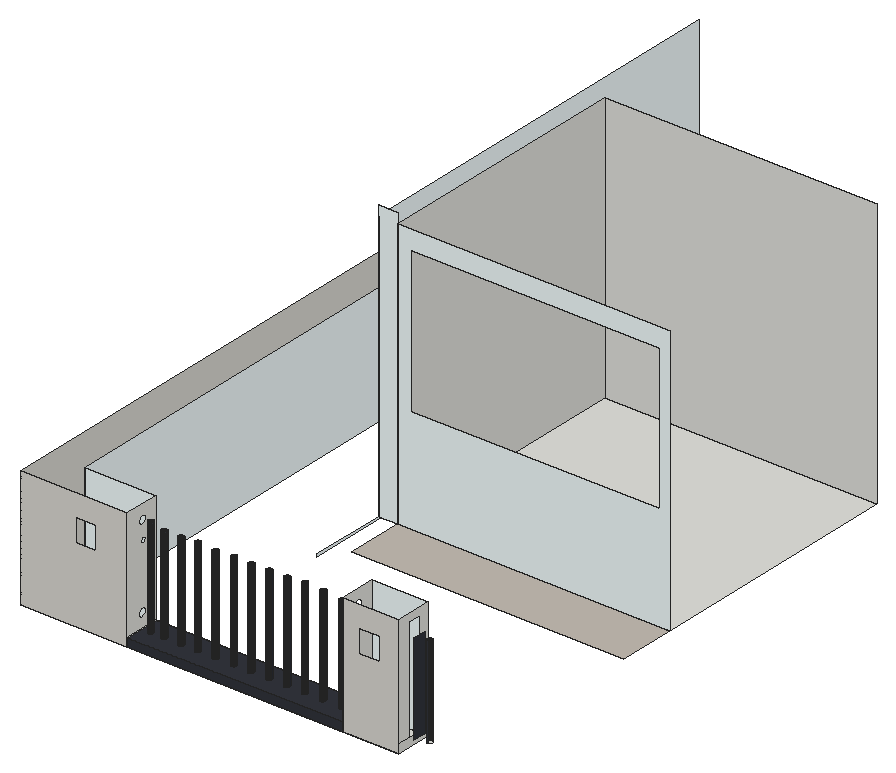
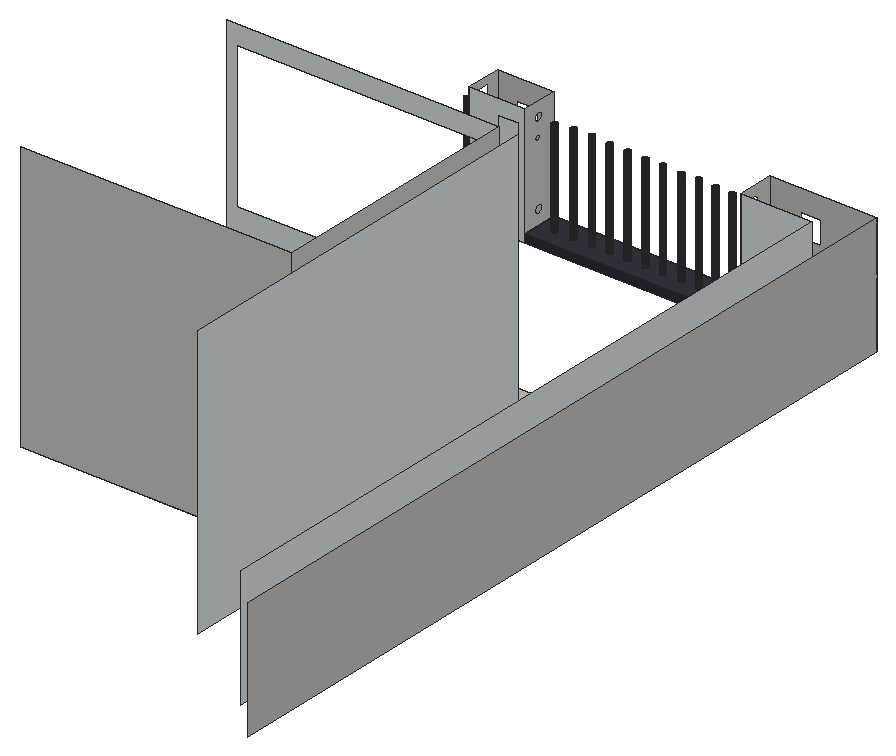
# SketchUp Ruby script. Lengths in inches.
U = 1.inch
M = Sketchup.active_model
def pt(a) = Geom::Point3d.new(a.map { |v| v * U })
def face(e, loops, mat)
  f = e.add_face(loops[0].map { |a| pt(a) })
  loops[1..].each { |l| e.add_face(l.map { |a| pt(a) }).erase! }
  f.material = f.back_material = mat if mat
  f
end
# faces: each face lists its corners as indices into pts; further lists are holes
def faces(e, pts, list, mat = nil) = list.each { |f| face(e, (f[0].is_a?(Array) ? f : [f]).map { |l| l.map { |i| pts[i] } }, mat) }
# xy, xz, yz: faces in a plane at the given z, y or x. An outline is a flat list of corners, or four numbers for a rectangle; further outlines are holes
def ring(l) = l.size == 4 ? [[l[0], l[1]], [l[2], l[1]], [l[2], l[3]], [l[0], l[3]]] : l.each_slice(2).to_a
def flat(e, list, mat, &to3) = list.each { |f| face(e, (f[0].is_a?(Array) ? f : [f]).map { |l| ring(l).map { |u, v| to3.(u, v) } }, mat) }
def xy(e, z, list, mat = nil) = flat(e, list, mat) { |x, y| [x, y, z] }
def xz(e, y, list, mat = nil) = flat(e, list, mat) { |x, z| [x, y, z] }
def yz(e, x, list, mat = nil) = flat(e, list, mat) { |y, z| [x, y, z] }
def lines(e, pts, list) = list.each { |a, b| e.add_line(pt(pts[a]), pt(pts[b])) }
# prism: a flat outline (further loops are holes) pulled along v
def prism(e, loops, v, mat = nil)
  f = face(e, loops, mat); d = Geom::Vector3d.new(v.map { |x| x * U })
  f.pushpull(f.normal.samedirection?(d) ? d.length : -d.length)
end
def box(e, o, s, mat = nil) = prism(e, [[o, [o[0] + s[0], o[1], o[2]], [o[0] + s[0], o[1] + s[1], o[2]], [o[0], o[1] + s[1], o[2]]]], [0, 0, s[2]], mat)
def at(x, y, z, deg = 0) = Geom::Transformation.translation(pt([x, y, z])) * Geom::Transformation.rotation(ORIGIN, Z_AXIS, deg.degrees)
def axes(o, x, y, z) = Geom::Transformation.new([*x, 0, *y, 0, *z, 0, *pt(o).to_a, 1])
def part(name) = M.definitions.add(name)
# library, detail: a bought-in or finely detailed component or shape, given as its bounding box
def library(name, o, s) = part(name).tap { |d| box(d.entities, o, s) }
def detail(e, o, s) = box(e.add_group.entities, o, s)
def put(e, d, t, mat = nil) = e.add_instance(d, t).tap { |i| i.material = mat if mat }
def group(e, t, mat = nil) = e.add_group.tap { |g| g.transformation = t; g.material = mat if mat }.entities
root = M.entities
M.materials.add("[Field Rectangle Tile]").color = [196, 189, 179]
M.materials.add("[Formica Laminate Dark]1").color = [50, 53, 60]
M.materials.add("[Terrazzo Tile Light]").color = [219, 217, 210]
M.materials.add("[White Subway Tile]").color = [243, 252, 253]
M.materials.add("[White Subway Tile]1").color = [243, 252, 253]
xy(root,0,[[383.65,0,1157.35,129.42],[1157.35,0,1357.59,129.42]])
xy(root,9,[[547.35,1008.89,1522.59,1933.89]])
xy(root,9,[[547.35,803.71,1522.59,1008.89]],"[Field Rectangle Tile]")
xy(root,29.875,[[416.3,55.58,413.8,55.72,411.41,56.51,409.31,57.89,407.64,59.76,406.51,62.01,405.99,64.47,406.14,66.98,406.92,69.36,408.3,71.46,410.18,73.14,412.42,74.27,414.88,74.78,417.39,74.64,419.77,73.85,421.875,72.47,423.55,70.6,424.68,68.35,425.19,65.89,425.05,63.38,424.26,61,422.88,58.9,421.01,57.22,418.76,56.09],[465.05,55.58,462.55,55.72,460.16,56.51,458.06,57.89,456.39,59.76,455.26,62.01,454.74,64.47,454.89,66.98,455.67,69.36,457.05,71.46,458.93,73.14,461.17,74.27,463.63,74.78,466.14,74.64,468.52,73.85,470.625,72.47,472.3,70.6,473.43,68.35,473.94,65.89,473.8,63.38,473.01,61,471.63,58.9,469.76,57.22,467.51,56.09],[525.12,55.58,522.61,55.72,520.22,56.51,518.12,57.89,516.45,59.76,515.32,62.01,514.81,64.47,514.95,66.98,515.74,69.36,517.11,71.46,518.99,73.14,521.23,74.27,523.69,74.78,526.2,74.64,528.59,73.85,530.6875,72.47,532.36,70.6,533.49,68.35,534,65.89,533.86,63.38,533.07,61,531.7,58.9,529.82,57.22,527.58,56.09],[585.24,55.58,582.73,55.72,580.35,56.51,578.25,57.89,576.57,59.76,575.44,62.01,574.93,64.47,575.07,66.98,575.86,69.36,577.24,71.46,579.11,73.14,581.36,74.27,583.82,74.78,586.33,74.64,588.71,73.85,590.8125,72.47,592.49,70.6,593.62,68.35,594.13,65.89,593.99,63.38,593.2,61,591.82,58.9,589.95,57.22,587.7,56.09],[648.8,55.58,646.3,55.72,643.91,56.51,641.81,57.89,640.14,59.76,639.01,62.01,638.49,64.47,638.64,66.98,639.42,69.36,640.8,71.46,642.68,73.14,644.92,74.27,647.38,74.78,649.89,74.64,652.27,73.85,654.375,72.47,656.05,70.6,657.18,68.35,657.69,65.89,657.55,63.38,656.76,61,655.38,58.9,653.51,57.22,651.26,56.09],
  [714.12,55.58,711.61,55.72,709.22,56.51,707.12,57.89,705.45,59.76,704.32,62.01,703.81,64.47,703.95,66.98,704.74,69.36,706.11,71.46,707.99,73.14,710.23,74.27,712.69,74.78,715.2,74.64,717.59,73.85,719.6875,72.47,721.36,70.6,722.49,68.35,723,65.89,722.86,63.38,722.07,61,720.7,58.9,718.82,57.22,716.58,56.09],[777.12,55.58,774.61,55.72,772.22,56.51,770.12,57.89,768.45,59.76,767.32,62.01,766.81,64.47,766.95,66.98,767.74,69.36,769.11,71.46,770.99,73.14,773.23,74.27,775.69,74.78,778.2,74.64,780.59,73.85,782.6875,72.47,784.36,70.6,785.49,68.35,786,65.89,785.86,63.38,785.07,61,783.7,58.9,781.82,57.22,779.58,56.09],[840.24,55.58,837.73,55.72,835.35,56.51,833.25,57.89,831.57,59.76,830.44,62.01,829.93,64.47,830.07,66.98,830.86,69.36,832.24,71.46,834.11,73.14,836.36,74.27,838.82,74.78,841.33,74.64,843.71,73.85,845.8125,72.47,847.49,70.6,848.62,68.35,849.13,65.89,848.99,63.38,848.2,61,846.82,58.9,844.95,57.22,842.7,56.09],[905.18,55.58,902.67,55.72,900.29,56.51,898.18,57.89,896.51,59.76,895.38,62.01,894.87,64.47,895.01,66.98,895.8,69.36,897.18,71.46,899.05,73.14,901.29,74.27,903.75,74.78,906.26,74.64,908.65,73.85,910.75,72.47,912.42,70.6,913.55,68.35,914.07,65.89,913.92,63.38,913.14,61,911.76,58.9,909.88,57.22,907.64,56.09],[968.99,55.58,966.48,55.72,964.1,56.51,962,57.89,960.32,59.76,959.19,62.01,958.68,64.47,958.82,66.98,959.61,69.36,960.99,71.46,962.86,73.14,965.11,74.27,967.57,74.78,970.08,74.64,972.46,73.85,974.5625,72.47,976.24,70.6,977.37,68.35,977.88,65.89,977.74,63.38,976.95,61,975.57,58.9,973.7,57.22,971.45,56.09],
  [1034.62,55.58,1032.11,55.72,1029.72,56.51,1027.62,57.89,1025.95,59.76,1024.82,62.01,1024.31,64.47,1024.45,66.98,1025.24,69.36,1026.61,71.46,1028.49,73.14,1030.73,74.27,1033.19,74.78,1035.7,74.64,1038.09,73.85,1040.1875,72.47,1041.86,70.6,1042.99,68.35,1043.5,65.89,1043.36,63.38,1042.57,61,1041.2,58.9,1039.32,57.22,1037.08,56.09],[1102.12,55.58,1099.61,55.72,1097.22,56.51,1095.12,57.89,1093.45,59.76,1092.32,62.01,1091.81,64.47,1091.95,66.98,1092.74,69.36,1094.11,71.46,1095.99,73.14,1098.23,74.27,1100.69,74.78,1103.2,74.64,1105.59,73.85,1107.6875,72.47,1109.36,70.6,1110.49,68.35,1111,65.89,1110.86,63.38,1110.07,61,1108.7,58.9,1106.82,57.22,1104.58,56.09],[1417.24,55.58,1414.73,55.72,1412.35,56.51,1410.25,57.89,1408.57,59.76,1407.44,62.01,1406.93,64.47,1407.07,66.98,1407.86,69.36,1409.24,71.46,1411.11,73.14,1413.36,74.27,1415.82,74.78,1418.33,74.64,1420.71,73.85,1422.8125,72.47,1424.49,70.6,1425.62,68.35,1426.13,65.89,1425.99,63.38,1425.2,61,1423.82,58.9,1421.95,57.22,1419.7,56.09]])
xy(root,29.875,[[[383.65,0,1157.35,129.42],[777.12,55.58,774.61,55.72,772.22,56.51,770.12,57.89,768.45,59.76,767.32,62.01,766.81,64.47,766.95,66.98,767.74,69.36,769.11,71.46,770.99,73.14,773.23,74.27,775.69,74.78,778.2,74.64,780.59,73.85,782.6875,72.47,784.36,70.6,785.49,68.35,786,65.89,785.86,63.38,785.07,61,783.7,58.9,781.82,57.22,779.58,56.09],[1102.12,55.58,1099.61,55.72,1097.22,56.51,1095.12,57.89,1093.45,59.76,1092.32,62.01,1091.81,64.47,1091.95,66.98,1092.74,69.36,1094.11,71.46,1095.99,73.14,1098.23,74.27,1100.69,74.78,1103.2,74.64,1105.59,73.85,1107.6875,72.47,1109.36,70.6,1110.49,68.35,1111,65.89,1110.86,63.38,1110.07,61,1108.7,58.9,1106.82,57.22,1104.58,56.09],[840.24,55.58,837.73,55.72,835.35,56.51,833.25,57.89,831.57,59.76,830.44,62.01,829.93,64.47,830.07,66.98,830.86,69.36,832.24,71.46,834.11,73.14,836.36,74.27,838.82,74.78,841.33,74.64,843.71,73.85,845.8125,72.47,847.49,70.6,848.62,68.35,849.13,65.89,848.99,63.38,848.2,61,846.82,58.9,844.95,57.22,842.7,56.09],[1034.62,55.58,1032.11,55.72,1029.72,56.51,1027.62,57.89,1025.95,59.76,1024.82,62.01,1024.31,64.47,1024.45,66.98,1025.24,69.36,1026.61,71.46,1028.49,73.14,1030.73,74.27,1033.19,74.78,1035.7,74.64,1038.09,73.85,1040.1875,72.47,1041.86,70.6,1042.99,68.35,1043.5,65.89,1043.36,63.38,1042.57,61,1041.2,58.9,1039.32,57.22,1037.08,56.09],[905.18,55.58,902.67,55.72,900.29,56.51,898.18,57.89,896.51,59.76,895.38,62.01,894.87,64.47,895.01,66.98,895.8,69.36,897.18,71.46,899.05,73.14,901.29,74.27,903.75,74.78,906.26,74.64,908.65,73.85,910.75,72.47,912.42,70.6,913.55,68.35,914.07,65.89,913.92,63.38,913.14,61,911.76,58.9,909.88,57.22,907.64,56.09],[968.99,55.58,966.48,55.72,964.1,56.51,962,57.89,960.32,59.76,959.19,62.01,958.68,64.47,958.82,66.98,959.61,69.36,960.99,71.46,962.86,73.14,965.11,74.27,967.57,74.78,970.08,74.64,972.46,73.85,974.5625,72.47,976.24,70.6,977.37,68.35,977.88,65.89,977.74,63.38,976.95,61,975.57,58.9,973.7,57.22,971.45,56.09],[416.3,55.58,413.8,55.72,411.41,56.51,409.31,57.89,407.64,59.76,406.51,62.01,405.99,64.47,406.14,66.98,406.92,69.36,408.3,71.46,410.18,73.14,412.42,74.27,414.88,74.78,417.39,74.64,419.77,73.85,421.875,72.47,423.55,70.6,424.68,68.35,425.19,65.89,425.05,63.38,424.26,61,422.88,58.9,421.01,57.22,418.76,56.09],[714.12,55.58,711.61,55.72,709.22,56.51,707.12,57.89,705.45,59.76,704.32,62.01,703.81,64.47,703.95,66.98,704.74,69.36,706.11,71.46,707.99,73.14,710.23,74.27,712.69,74.78,715.2,74.64,717.59,73.85,719.6875,72.47,721.36,70.6,722.49,68.35,723,65.89,722.86,63.38,722.07,61,720.7,58.9,718.82,57.22,716.58,56.09],[465.05,55.58,462.55,55.72,460.16,56.51,458.06,57.89,456.39,59.76,455.26,62.01,454.74,64.47,454.89,66.98,455.67,69.36,457.05,71.46,458.93,73.14,461.17,74.27,463.63,74.78,466.14,74.64,468.52,73.85,470.625,72.47,472.3,70.6,473.43,68.35,473.94,65.89,473.8,63.38,473.01,61,471.63,58.9,469.76,57.22,467.51,56.09],[648.8,55.58,646.3,55.72,643.91,56.51,641.81,57.89,640.14,59.76,639.01,62.01,638.49,64.47,638.64,66.98,639.42,69.36,640.8,71.46,642.68,73.14,644.92,74.27,647.38,74.78,649.89,74.64,652.27,73.85,654.375,72.47,656.05,70.6,657.18,68.35,657.69,65.89,657.55,63.38,656.76,61,655.38,58.9,653.51,57.22,651.26,56.09],[525.12,55.58,522.61,55.72,520.22,56.51,518.12,57.89,516.45,59.76,515.32,62.01,514.81,64.47,514.95,66.98,515.74,69.36,517.11,71.46,518.99,73.14,521.23,74.27,523.69,74.78,526.2,74.64,528.59,73.85,530.6875,72.47,532.36,70.6,533.49,68.35,534,65.89,533.86,63.38,533.07,61,531.7,58.9,529.82,57.22,527.58,56.09],[585.24,55.58,582.73,55.72,580.35,56.51,578.25,57.89,576.57,59.76,575.44,62.01,574.93,64.47,575.07,66.98,575.86,69.36,577.24,71.46,579.11,73.14,581.36,74.27,583.82,74.78,586.33,74.64,588.71,73.85,590.8125,72.47,592.49,70.6,593.62,68.35,594.13,65.89,593.99,63.38,593.2,61,591.82,58.9,589.95,57.22,587.7,56.09]]],"[Formica Laminate Dark]1")
xz(root,0,[[383.65,0,1157.35,29.875]],"[Formica Laminate Dark]1")
xz(root,0,[[[0,0,383.65,429.3125],[199.14,268.73,272.27,354.42]],[[1157.35,0,1357.59,429.3125],[1214.39,268.73,1287.52,354.42]]],"[Terrazzo Tile Light]")
xz(root,129.42,[[383.65,0,1157.35,29.875]],"[Formica Laminate Dark]1")
xz(root,129.42,[[129.42,0,383.65,429.3125],[1157.35,0,1357.59,429.3125]],"[White Subway Tile]1")
xz(root,1008.89,[[477.43,9,547.35,1009.375],[[547.35,9,1522.59,973.375],[594.7,387.41,1485.01,905.79]]],"[White Subway Tile]")
xz(root,1933.89,[[547.35,9,1522.59,973.375]])
yz(root,0,[[0,0,2816.0625,429.3125]],"[Terrazzo Tile Light]")
yz(root,129.42,[[129.42,0,2686.64,429.3125]],"[White Subway Tile]1")
yz(root,383.65,[[0,0,129.42,29.875],[[0,29.875,129.42,429.3125],[67.74,66.35,63.84,66.87,60.21,68.37,57.09,70.76,54.7,73.88,53.19,77.52,52.68,81.42,53.19,85.3125,54.7,88.95,57.09,92.07,60.21,94.46,63.84,95.96,67.74,96.48,71.64,95.96,75.27,94.46,78.39,92.07,80.79,88.95,82.29,85.3125,82.81,81.42,82.29,77.52,80.79,73.88,78.39,70.76,75.27,68.37,71.64,66.87],[67.74,363.79,63.84,364.3,60.21,365.81,57.09,368.2,54.7,371.32,53.19,374.95,52.68,378.85,53.19,382.75,54.7,386.38,57.09,389.5,60.21,391.9,63.84,393.4,67.74,393.92,71.64,393.4,75.27,391.9,78.39,389.5,80.79,386.38,82.29,382.75,82.81,378.85,82.29,374.95,80.79,371.32,78.39,368.2,75.27,365.81,71.64,364.3],[71.79,301.92,69.12,302.27,66.63,303.3,64.5,304.9375,62.86,307.07,61.83,309.5625,61.48,312.23,61.83,314.9,62.86,317.39,64.5,319.52,66.63,321.16,69.12,322.19,71.79,322.54,74.46,322.19,76.94,321.16,79.08,319.52,80.72,317.39,81.75,314.9,82.1,312.23,81.75,309.5625,80.72,307.07,79.08,304.9375,76.94,303.3,74.46,302.27]]])
yz(root,477.43,[[733.79,0,733.79,9,1008.89,9,1008.89,973.375,2442.87,973.375,2442.87,0]],"[White Subway Tile]")
yz(root,547.35,[[1008.89,9,1933.89,973.375]])
yz(root,1157.35,[[0,0,129.42,29.875],[[0,29.875,129.42,429.3125],[67.74,363.79,71.64,364.3,75.27,365.81,78.39,368.2,80.79,371.32,82.29,374.95,82.81,378.85,82.29,382.75,80.79,386.38,78.39,389.5,75.27,391.9,71.64,393.4,67.74,393.92,63.84,393.4,60.21,391.9,57.09,389.5,54.7,386.38,53.19,382.75,52.68,378.85,53.19,374.95,54.7,371.32,57.09,368.2,60.21,365.81,63.84,364.3],[67.74,66.35,71.64,66.87,75.27,68.37,78.39,70.76,80.79,73.88,82.29,77.52,82.81,81.42,82.29,85.3125,80.79,88.95,78.39,92.07,75.27,94.46,71.64,95.96,67.74,96.48,63.84,95.96,60.21,94.46,57.09,92.07,54.7,88.95,53.19,85.3125,52.68,81.42,53.19,77.52,54.7,73.88,57.09,70.76,60.21,68.37,63.84,66.87],[71.79,301.92,74.46,302.27,76.94,303.3,79.08,304.9375,80.72,307.07,81.75,309.5625,82.1,312.23,81.75,314.9,80.72,317.39,79.08,319.52,76.94,321.16,74.46,322.19,71.79,322.54,69.12,322.19,66.63,321.16,64.5,319.52,62.86,317.39,61.83,314.9,61.48,312.23,61.83,309.5625,62.86,307.07,64.5,304.9375,66.63,303.3,69.12,302.27]]])
yz(root,1357.59,[[0,0,129.42,29.875],[0,29.875,44.85,29.875,44.85,402.23,92.78,402.23,92.78,29.875,129.42,29.875,129.42,429.3125,0,429.3125]])
yz(root,1376.86,[[44.85,29.875,92.78,357.02]],"[Formica Laminate Dark]1")
p = [[413.8,55.72,29.875],[416.3,55.58,29.875],[416.3,55.58,386.38],[413.8,55.72,386.38],[418.76,56.09,29.875],[418.76,56.09,386.38],
  [462.55,55.72,29.875],[465.05,55.58,29.875],[465.05,55.58,373.4375],[462.55,55.72,373.4375],[467.51,56.09,29.875],[467.51,56.09,373.4375],
  [522.61,55.72,29.875],[525.12,55.58,29.875],[525.12,55.58,374.6875],[522.61,55.72,374.6875],[527.58,56.09,29.875],[527.58,56.09,374.6875],
  [582.73,55.72,29.875],[585.24,55.58,29.875],[585.24,55.58,378.85],[582.73,55.72,378.85],[587.7,56.09,29.875],[587.7,56.09,378.85],
  [646.3,55.72,29.875],[648.8,55.58,29.875],[648.8,55.58,374.5625],[646.3,55.72,374.5625],[651.26,56.09,29.875],[651.26,56.09,374.5625],
  [711.61,55.72,29.875],[714.12,55.58,29.875],[714.12,55.58,378.25],[711.61,55.72,378.25],[716.58,56.09,29.875],[716.58,56.09,378.25],
  [774.61,55.72,29.875],[777.12,55.58,29.875],[777.12,55.58,376.5],[774.61,55.72,376.5],[779.58,56.09,29.875],[779.58,56.09,376.5],
  [837.73,55.72,29.875],[840.24,55.58,29.875],[840.24,55.58,378.85],[837.73,55.72,378.85],[842.7,56.09,29.875],[842.7,56.09,378.85],
  [902.67,55.72,29.875],[905.18,55.58,29.875],[905.18,55.58,379.125],[902.67,55.72,379.125],[907.64,56.09,29.875],[907.64,56.09,379.125],
  [966.48,55.72,29.875],[968.99,55.58,29.875],[968.99,55.58,384.0625],[966.48,55.72,384.0625],[971.45,56.09,29.875],[971.45,56.09,384.0625],
  [1032.11,55.72,29.875],[1034.62,55.58,29.875],[1034.62,55.58,381.875],[1032.11,55.72,381.875],[1037.08,56.09,29.875],[1037.08,56.09,381.875],
  [1099.61,55.72,29.875],[1102.12,55.58,29.875],[1102.12,55.58,375.0625],[1099.61,55.72,375.0625],[1104.58,56.09,29.875],[1104.58,56.09,375.0625],
  [1414.73,55.72,29.875],[1417.24,55.58,29.875],[1417.24,55.58,357.02],[1414.73,55.72,357.02],[411.41,56.51,29.875],[411.41,56.51,386.38],
  [460.16,56.51,29.875],[460.16,56.51,373.4375],[520.22,56.51,29.875],[520.22,56.51,374.6875],[580.35,56.51,29.875],[580.35,56.51,378.85],
  [643.91,56.51,29.875],[643.91,56.51,374.5625],[709.22,56.51,29.875],[709.22,56.51,378.25],[772.22,56.51,29.875],[772.22,56.51,376.5],
  [835.35,56.51,29.875],[835.35,56.51,378.85],[900.29,56.51,29.875],[900.29,56.51,379.125],[964.1,56.51,29.875],[964.1,56.51,384.0625],
  [1029.72,56.51,29.875],[1029.72,56.51,381.875],[1097.22,56.51,29.875],[1097.22,56.51,375.0625],[1412.35,56.51,29.875],[1412.35,56.51,357.02],
  [421.01,57.22,29.875],[421.01,57.22,386.38],[469.76,57.22,29.875],[469.76,57.22,373.4375],[529.82,57.22,29.875],[529.82,57.22,374.6875],
  [589.95,57.22,29.875],[589.95,57.22,378.85],[653.51,57.22,29.875],[653.51,57.22,374.5625],[718.82,57.22,29.875],[718.82,57.22,378.25],
  [781.82,57.22,29.875],[781.82,57.22,376.5],[844.95,57.22,29.875],[844.95,57.22,378.85],[909.88,57.22,29.875],[909.88,57.22,379.125],
  [973.7,57.22,29.875],[973.7,57.22,384.0625],[1039.32,57.22,29.875],[1039.32,57.22,381.875],[1106.82,57.22,29.875],[1106.82,57.22,375.0625],
  [409.31,57.89,29.875],[409.31,57.89,386.38],[458.06,57.89,29.875],[458.06,57.89,373.4375],[518.12,57.89,29.875],[518.12,57.89,374.6875],
  [578.25,57.89,29.875],[578.25,57.89,378.85],[641.81,57.89,29.875],[641.81,57.89,374.5625],[707.12,57.89,29.875],[707.12,57.89,378.25],
  [770.12,57.89,29.875],[770.12,57.89,376.5],[833.25,57.89,29.875],[833.25,57.89,378.85],[898.18,57.89,29.875],[898.18,57.89,379.125],
  [962,57.89,29.875],[962,57.89,384.0625],[1027.62,57.89,29.875],[1027.62,57.89,381.875],[1095.12,57.89,29.875],[1095.12,57.89,375.0625],
  [1410.25,57.89,29.875],[1410.25,57.89,357.02],[422.88,58.9,29.875],[422.88,58.9,386.38],[471.63,58.9,29.875],[471.63,58.9,373.4375],
  [531.7,58.9,29.875],[531.7,58.9,374.6875],[591.82,58.9,29.875],[591.82,58.9,378.85],[655.38,58.9,29.875],[655.38,58.9,374.5625],
  [720.7,58.9,29.875],[720.7,58.9,378.25],[783.7,58.9,29.875],[783.7,58.9,376.5],[846.82,58.9,29.875],[846.82,58.9,378.85],
  [911.76,58.9,29.875],[911.76,58.9,379.125],[975.57,58.9,29.875],[975.57,58.9,384.0625],[1041.2,58.9,29.875],[1041.2,58.9,381.875],
  [1108.7,58.9,29.875],[1108.7,58.9,375.0625],[407.64,59.76,29.875],[407.64,59.76,386.38],[456.39,59.76,29.875],[456.39,59.76,373.4375],
  [516.45,59.76,29.875],[516.45,59.76,374.6875],[576.57,59.76,29.875],[576.57,59.76,378.85],[640.14,59.76,29.875],[640.14,59.76,374.5625],
  [705.45,59.76,29.875],[705.45,59.76,378.25],[768.45,59.76,29.875],[768.45,59.76,376.5],[831.57,59.76,29.875],[831.57,59.76,378.85],
  [896.51,59.76,29.875],[896.51,59.76,379.125],[960.32,59.76,29.875],[960.32,59.76,384.0625],[1025.95,59.76,29.875],[1025.95,59.76,381.875],
  [1093.45,59.76,29.875],[1093.45,59.76,375.0625],[1408.57,59.76,29.875],[1408.57,59.76,357.02],[424.26,61,29.875],[424.26,61,386.38],
  [473.01,61,29.875],[473.01,61,373.4375],[533.07,61,29.875],[533.07,61,374.6875],[593.2,61,29.875],[593.2,61,378.85],
  [656.76,61,29.875],[656.76,61,374.5625],[722.07,61,29.875],[722.07,61,378.25],[785.07,61,29.875],[785.07,61,376.5],
  [848.2,61,29.875],[848.2,61,378.85],[913.14,61,29.875],[913.14,61,379.125],[976.95,61,29.875],[976.95,61,384.0625],
  [1042.57,61,29.875],[1042.57,61,381.875],[1110.07,61,29.875],[1110.07,61,375.0625],[406.51,62.01,29.875],[406.51,62.01,386.38],
  [455.26,62.01,29.875],[455.26,62.01,373.4375],[515.32,62.01,29.875],[515.32,62.01,374.6875],[575.44,62.01,29.875],[575.44,62.01,378.85],
  [639.01,62.01,29.875],[639.01,62.01,374.5625],[704.32,62.01,29.875],[704.32,62.01,378.25],[767.32,62.01,29.875],[767.32,62.01,376.5],
  [830.44,62.01,29.875],[830.44,62.01,378.85],[895.38,62.01,29.875],[895.38,62.01,379.125],[959.19,62.01,29.875],[959.19,62.01,384.0625],
  [1024.82,62.01,29.875],[1024.82,62.01,381.875],[1092.32,62.01,29.875],[1092.32,62.01,375.0625],[1407.44,62.01,29.875],[1407.44,62.01,357.02],
  [425.05,63.38,29.875],[425.05,63.38,386.38],[473.8,63.38,29.875],[473.8,63.38,373.4375],[533.86,63.38,29.875],[533.86,63.38,374.6875],
  [593.99,63.38,29.875],[593.99,63.38,378.85],[657.55,63.38,29.875],[657.55,63.38,374.5625],[722.86,63.38,29.875],[722.86,63.38,378.25],
  [785.86,63.38,29.875],[785.86,63.38,376.5],[848.99,63.38,29.875],[848.99,63.38,378.85],[913.92,63.38,29.875],[913.92,63.38,379.125],
  [977.74,63.38,29.875],[977.74,63.38,384.0625],[1043.36,63.38,29.875],[1043.36,63.38,381.875],[1110.86,63.38,29.875],[1110.86,63.38,375.0625],
  [405.99,64.47,29.875],[405.99,64.47,386.38],[454.74,64.47,29.875],[454.74,64.47,373.4375],[514.81,64.47,29.875],[514.81,64.47,374.6875],
  [574.93,64.47,29.875],[574.93,64.47,378.85],[638.49,64.47,29.875],[638.49,64.47,374.5625],[703.81,64.47,29.875],[703.81,64.47,378.25],
  [766.81,64.47,29.875],[766.81,64.47,376.5],[829.93,64.47,29.875],[829.93,64.47,378.85],[894.87,64.47,29.875],[894.87,64.47,379.125],
  [958.68,64.47,29.875],[958.68,64.47,384.0625],[1024.31,64.47,29.875],[1024.31,64.47,381.875],[1091.81,64.47,29.875],[1091.81,64.47,375.0625],
  [1406.93,64.47,29.875],[1406.93,64.47,357.02],[425.19,65.89,29.875],[425.19,65.89,386.38],[473.94,65.89,29.875],[473.94,65.89,373.4375],
  [534,65.89,29.875],[534,65.89,374.6875],[594.13,65.89,29.875],[594.13,65.89,378.85],[657.69,65.89,29.875],[657.69,65.89,374.5625],
  [723,65.89,29.875],[723,65.89,378.25],[786,65.89,29.875],[786,65.89,376.5],[849.13,65.89,29.875],[849.13,65.89,378.85],
  [914.07,65.89,29.875],[914.07,65.89,379.125],[977.88,65.89,29.875],[977.88,65.89,384.0625],[1043.5,65.89,29.875],[1043.5,65.89,381.875],
  [1111,65.89,29.875],[1111,65.89,375.0625],[406.14,66.98,29.875],[406.14,66.98,386.38],[454.89,66.98,29.875],[454.89,66.98,373.4375],
  [514.95,66.98,29.875],[514.95,66.98,374.6875],[575.07,66.98,29.875],[575.07,66.98,378.85],[638.64,66.98,29.875],[638.64,66.98,374.5625],
  [703.95,66.98,29.875],[703.95,66.98,378.25],[766.95,66.98,29.875],[766.95,66.98,376.5],[830.07,66.98,29.875],[830.07,66.98,378.85],
  [895.01,66.98,29.875],[895.01,66.98,379.125],[958.82,66.98,29.875],[958.82,66.98,384.0625],[1024.45,66.98,29.875],[1024.45,66.98,381.875],
  [1091.95,66.98,29.875],[1091.95,66.98,375.0625],[1407.07,66.98,29.875],[1407.07,66.98,357.02],[424.68,68.35,29.875],[424.68,68.35,386.38],
  [473.43,68.35,29.875],[473.43,68.35,373.4375],[533.49,68.35,29.875],[533.49,68.35,374.6875],[593.62,68.35,29.875],[593.62,68.35,378.85],
  [657.18,68.35,29.875],[657.18,68.35,374.5625],[722.49,68.35,29.875],[722.49,68.35,378.25],[785.49,68.35,29.875],[785.49,68.35,376.5],
  [848.62,68.35,29.875],[848.62,68.35,378.85],[913.55,68.35,29.875],[913.55,68.35,379.125],[977.37,68.35,29.875],[977.37,68.35,384.0625],
  [1042.99,68.35,29.875],[1042.99,68.35,381.875],[1110.49,68.35,29.875],[1110.49,68.35,375.0625],[406.92,69.36,29.875],[406.92,69.36,386.38],
  [455.67,69.36,29.875],[455.67,69.36,373.4375],[515.74,69.36,29.875],[515.74,69.36,374.6875],[575.86,69.36,29.875],[575.86,69.36,378.85],
  [639.42,69.36,29.875],[639.42,69.36,374.5625],[704.74,69.36,29.875],[704.74,69.36,378.25],[767.74,69.36,29.875],[767.74,69.36,376.5],
  [830.86,69.36,29.875],[830.86,69.36,378.85],[895.8,69.36,29.875],[895.8,69.36,379.125],[959.61,69.36,29.875],[959.61,69.36,384.0625],
  [1025.24,69.36,29.875],[1025.24,69.36,381.875],[1092.74,69.36,29.875],[1092.74,69.36,375.0625],[1407.86,69.36,29.875],[1407.86,69.36,357.02],
  [423.55,70.6,29.875],[423.55,70.6,386.38],[472.3,70.6,29.875],[472.3,70.6,373.4375],[532.36,70.6,29.875],[532.36,70.6,374.6875],
  [592.49,70.6,29.875],[592.49,70.6,378.85],[656.05,70.6,29.875],[656.05,70.6,374.5625],[721.36,70.6,29.875],[721.36,70.6,378.25],
  [784.36,70.6,29.875],[784.36,70.6,376.5],[847.49,70.6,29.875],[847.49,70.6,378.85],[912.42,70.6,29.875],[912.42,70.6,379.125],
  [976.24,70.6,29.875],[976.24,70.6,384.0625],[1041.86,70.6,29.875],[1041.86,70.6,381.875],[1109.36,70.6,29.875],[1109.36,70.6,375.0625],
  [408.3,71.46,29.875],[408.3,71.46,386.38],[457.05,71.46,29.875],[457.05,71.46,373.4375],[517.11,71.46,29.875],[517.11,71.46,374.6875],
  [577.24,71.46,29.875],[577.24,71.46,378.85],[640.8,71.46,29.875],[640.8,71.46,374.5625],[706.11,71.46,29.875],[706.11,71.46,378.25],
  [769.11,71.46,29.875],[769.11,71.46,376.5],[832.24,71.46,29.875],[832.24,71.46,378.85],[897.18,71.46,29.875],[897.18,71.46,379.125],
  [960.99,71.46,29.875],[960.99,71.46,384.0625],[1026.61,71.46,29.875],[1026.61,71.46,381.875],[1094.11,71.46,29.875],[1094.11,71.46,375.0625],
  [1409.24,71.46,29.875],[1409.24,71.46,357.02],[421.875,72.47,29.875],[421.875,72.47,386.38],[470.625,72.47,29.875],[470.625,72.47,373.4375],
  [530.6875,72.47,29.875],[530.6875,72.47,374.6875],[590.8125,72.47,29.875],[590.8125,72.47,378.85],[654.375,72.47,29.875],[654.375,72.47,374.5625],
  [719.6875,72.47,29.875],[719.6875,72.47,378.25],[782.6875,72.47,29.875],[782.6875,72.47,376.5],[845.8125,72.47,29.875],[845.8125,72.47,378.85],
  [910.75,72.47,29.875],[910.75,72.47,379.125],[974.5625,72.47,29.875],[974.5625,72.47,384.0625],[1040.1875,72.47,29.875],[1040.1875,72.47,381.875],
  [1107.6875,72.47,29.875],[1107.6875,72.47,375.0625],[410.18,73.14,29.875],[410.18,73.14,386.38],[458.93,73.14,29.875],[458.93,73.14,373.4375],
  [518.99,73.14,29.875],[518.99,73.14,374.6875],[579.11,73.14,29.875],[579.11,73.14,378.85],[642.68,73.14,29.875],[642.68,73.14,374.5625],
  [707.99,73.14,29.875],[707.99,73.14,378.25],[770.99,73.14,29.875],[770.99,73.14,376.5],[834.11,73.14,29.875],[834.11,73.14,378.85],
  [899.05,73.14,29.875],[899.05,73.14,379.125],[962.86,73.14,29.875],[962.86,73.14,384.0625],[1028.49,73.14,29.875],[1028.49,73.14,381.875],
  [1095.99,73.14,29.875],[1095.99,73.14,375.0625],[1411.11,73.14,29.875],[1411.11,73.14,357.02],[419.77,73.85,29.875],[419.77,73.85,386.38],
  [468.52,73.85,29.875],[468.52,73.85,373.4375],[528.59,73.85,29.875],[528.59,73.85,374.6875],[588.71,73.85,29.875],[588.71,73.85,378.85],
  [652.27,73.85,29.875],[652.27,73.85,374.5625],[717.59,73.85,29.875],[717.59,73.85,378.25],[780.59,73.85,29.875],[780.59,73.85,376.5],
  [843.71,73.85,29.875],[843.71,73.85,378.85],[908.65,73.85,29.875],[908.65,73.85,379.125],[972.46,73.85,29.875],[972.46,73.85,384.0625],
  [1038.09,73.85,29.875],[1038.09,73.85,381.875],[1105.59,73.85,29.875],[1105.59,73.85,375.0625],[412.42,74.27,29.875],[412.42,74.27,386.38],
  [461.17,74.27,29.875],[461.17,74.27,373.4375],[521.23,74.27,29.875],[521.23,74.27,374.6875],[581.36,74.27,29.875],[581.36,74.27,378.85],
  [644.92,74.27,29.875],[644.92,74.27,374.5625],[710.23,74.27,29.875],[710.23,74.27,378.25],[773.23,74.27,29.875],[773.23,74.27,376.5],
  [836.36,74.27,29.875],[836.36,74.27,378.85],[901.29,74.27,29.875],[901.29,74.27,379.125],[965.11,74.27,29.875],[965.11,74.27,384.0625],
  [1030.73,74.27,29.875],[1030.73,74.27,381.875],[1098.23,74.27,29.875],[1098.23,74.27,375.0625],[1413.36,74.27,29.875],[1413.36,74.27,357.02],
  [417.39,74.64,29.875],[417.39,74.64,386.38],[466.14,74.64,29.875],[466.14,74.64,373.4375],[526.2,74.64,29.875],[526.2,74.64,374.6875],
  [586.33,74.64,29.875],[586.33,74.64,378.85],[649.89,74.64,29.875],[649.89,74.64,374.5625],[715.2,74.64,29.875],[715.2,74.64,378.25],
  [778.2,74.64,29.875],[778.2,74.64,376.5],[841.33,74.64,29.875],[841.33,74.64,378.85],[906.26,74.64,29.875],[906.26,74.64,379.125],
  [970.08,74.64,29.875],[970.08,74.64,384.0625],[1035.7,74.64,29.875],[1035.7,74.64,381.875],[1103.2,74.64,29.875],[1103.2,74.64,375.0625],
  [414.88,74.78,29.875],[414.88,74.78,386.38],[463.63,74.78,29.875],[463.63,74.78,373.4375],[523.69,74.78,29.875],[523.69,74.78,374.6875],
  [583.82,74.78,29.875],[583.82,74.78,378.85],[647.38,74.78,29.875],[647.38,74.78,374.5625],[712.69,74.78,29.875],[712.69,74.78,378.25],
  [775.69,74.78,29.875],[775.69,74.78,376.5],[838.82,74.78,29.875],[838.82,74.78,378.85],[903.75,74.78,29.875],[903.75,74.78,379.125],
  [967.57,74.78,29.875],[967.57,74.78,384.0625],[1033.19,74.78,29.875],[1033.19,74.78,381.875],[1100.69,74.78,29.875],[1100.69,74.78,375.0625],
  [1415.82,74.78,29.875],[1415.82,74.78,357.02],[1418.33,74.64,29.875],[1418.33,74.64,357.02]]
faces(root,p,[[0,1,2,3],[1,4,5,2],[6,7,8,9],[7,10,11,8],[12,13,14,15],[13,16,17,14],[18,19,20,21],[19,22,23,20],
  [24,25,26,27],[25,28,29,26],[30,31,32,33],[31,34,35,32],[36,37,38,39],[37,40,41,38],[42,43,44,45],[43,46,47,44],
  [48,49,50,51],[49,52,53,50],[54,55,56,57],[55,58,59,56],[60,61,62,63],[61,64,65,62],[66,67,68,69],[67,70,71,68],
  [72,73,74,75],[76,0,3,77],[78,6,9,79],[80,12,15,81],[82,18,21,83],[84,24,27,85],[86,30,33,87],[88,36,39,89],
  [90,42,45,91],[92,48,51,93],[94,54,57,95],[96,60,63,97],[98,66,69,99],[100,72,75,101],[4,102,103,5],[10,104,105,11],
  [16,106,107,17],[22,108,109,23],[28,110,111,29],[34,112,113,35],[40,114,115,41],[46,116,117,47],[52,118,119,53],[58,120,121,59],
  [64,122,123,65],[70,124,125,71],[126,76,77,127],[128,78,79,129],[130,80,81,131],[132,82,83,133],[134,84,85,135],[136,86,87,137],
  [138,88,89,139],[140,90,91,141],[142,92,93,143],[144,94,95,145],[146,96,97,147],[148,98,99,149],[150,100,101,151],[102,152,153,103],
  [104,154,155,105],[106,156,157,107],[108,158,159,109],[110,160,161,111],[112,162,163,113],[114,164,165,115],[116,166,167,117],[118,168,169,119],
  [120,170,171,121],[122,172,173,123],[124,174,175,125],[176,126,127,177],[178,128,129,179],[180,130,131,181],[182,132,133,183],[184,134,135,185],
  [186,136,137,187],[188,138,139,189],[190,140,141,191],[192,142,143,193],[194,144,145,195],[196,146,147,197],[198,148,149,199],[200,150,151,201],
  [152,202,203,153],[154,204,205,155],[156,206,207,157],[158,208,209,159],[160,210,211,161],[162,212,213,163],[164,214,215,165],[166,216,217,167],
  [168,218,219,169],[170,220,221,171],[172,222,223,173],[174,224,225,175],[226,176,177,227],[228,178,179,229],[230,180,181,231],[232,182,183,233],
  [234,184,185,235],[236,186,187,237],[238,188,189,239],[240,190,191,241],[242,192,193,243],[244,194,195,245],[246,196,197,247],[248,198,199,249],
  [250,200,201,251],[202,252,253,203],[204,254,255,205],[206,256,257,207],[208,258,259,209],[210,260,261,211],[212,262,263,213],[214,264,265,215],
  [216,266,267,217],[218,268,269,219],[220,270,271,221],[222,272,273,223],[224,274,275,225],[276,226,227,277],[278,228,229,279],[280,230,231,281],
  [282,232,233,283],[284,234,235,285],[286,236,237,287],[288,238,239,289],[290,240,241,291],[292,242,243,293],[294,244,245,295],[296,246,247,297],
  [298,248,249,299],[300,250,251,301],[252,302,303,253],[254,304,305,255],[256,306,307,257],[258,308,309,259],[260,310,311,261],[262,312,313,263],
  [264,314,315,265],[266,316,317,267],[268,318,319,269],[270,320,321,271],[272,322,323,273],[274,324,325,275],[326,276,277,327],[328,278,279,329],
  [330,280,281,331],[332,282,283,333],[334,284,285,335],[336,286,287,337],[338,288,289,339],[340,290,291,341],[342,292,293,343],[344,294,295,345],
  [346,296,297,347],[348,298,299,349],[350,300,301,351],[302,352,353,303],[304,354,355,305],[306,356,357,307],[308,358,359,309],[310,360,361,311],
  [312,362,363,313],[314,364,365,315],[316,366,367,317],[318,368,369,319],[320,370,371,321],[322,372,373,323],[324,374,375,325],[376,326,327,377],
  [378,328,329,379],[380,330,331,381],[382,332,333,383],[384,334,335,385],[386,336,337,387],[388,338,339,389],[390,340,341,391],[392,342,343,393],
  [394,344,345,395],[396,346,347,397],[398,348,349,399],[400,350,351,401],[352,402,403,353],[354,404,405,355],[356,406,407,357],[358,408,409,359],
  [360,410,411,361],[362,412,413,363],[364,414,415,365],[366,416,417,367],[368,418,419,369],[370,420,421,371],[372,422,423,373],[374,424,425,375],
  [426,376,377,427],[428,378,379,429],[430,380,381,431],[432,382,383,433],[434,384,385,435],[436,386,387,437],[438,388,389,439],[440,390,391,441],
  [442,392,393,443],[444,394,395,445],[446,396,397,447],[448,398,399,449],[450,400,401,451],[402,452,453,403],[404,454,455,405],[406,456,457,407],
  [408,458,459,409],[410,460,461,411],[412,462,463,413],[414,464,465,415],[416,466,467,417],[418,468,469,419],[420,470,471,421],[422,472,473,423],
  [424,474,475,425],[476,426,427,477],[478,428,429,479],[480,430,431,481],[482,432,433,483],[484,434,435,485],[486,436,437,487],[488,438,439,489],
  [490,440,441,491],[492,442,443,493],[494,444,445,495],[496,446,447,497],[498,448,449,499],[500,450,451,501],[452,502,503,453],[454,504,505,455],
  [456,506,507,457],[458,508,509,459],[460,510,511,461],[462,512,513,463],[464,514,515,465],[466,516,517,467],[468,518,519,469],[470,520,521,471],
  [472,522,523,473],[474,524,525,475],[526,476,477,527],[528,478,479,529],[530,480,481,531],[532,482,483,533],[534,484,485,535],[536,486,487,537],
  [538,488,489,539],[540,490,491,541],[542,492,493,543],[544,494,495,545],[546,496,497,547],[548,498,499,549],[550,500,501,551],[502,552,553,503],
  [504,554,555,505],[506,556,557,507],[508,558,559,509],[510,560,561,511],[512,562,563,513],[514,564,565,515],[516,566,567,517],[518,568,569,519],
  [520,570,571,521],[522,572,573,523],[524,574,575,525],[576,526,527,577],[578,528,529,579],[580,530,531,581],[582,532,533,583],[584,534,535,585],
  [586,536,537,587],[588,538,539,589],[590,540,541,591],[592,542,543,593],[594,544,545,595],[596,546,547,597],[598,548,549,599],[600,550,551,601],
  [552,576,577,553],[554,578,579,555],[556,580,581,557],[558,582,583,559],[560,584,585,561],[562,586,587,563],[564,588,589,565],[566,590,591,567],
  [568,592,593,569],[570,594,595,571],[572,596,597,573],[574,598,599,575],[602,600,601,603]],"[Formica Laminate Dark]1")
